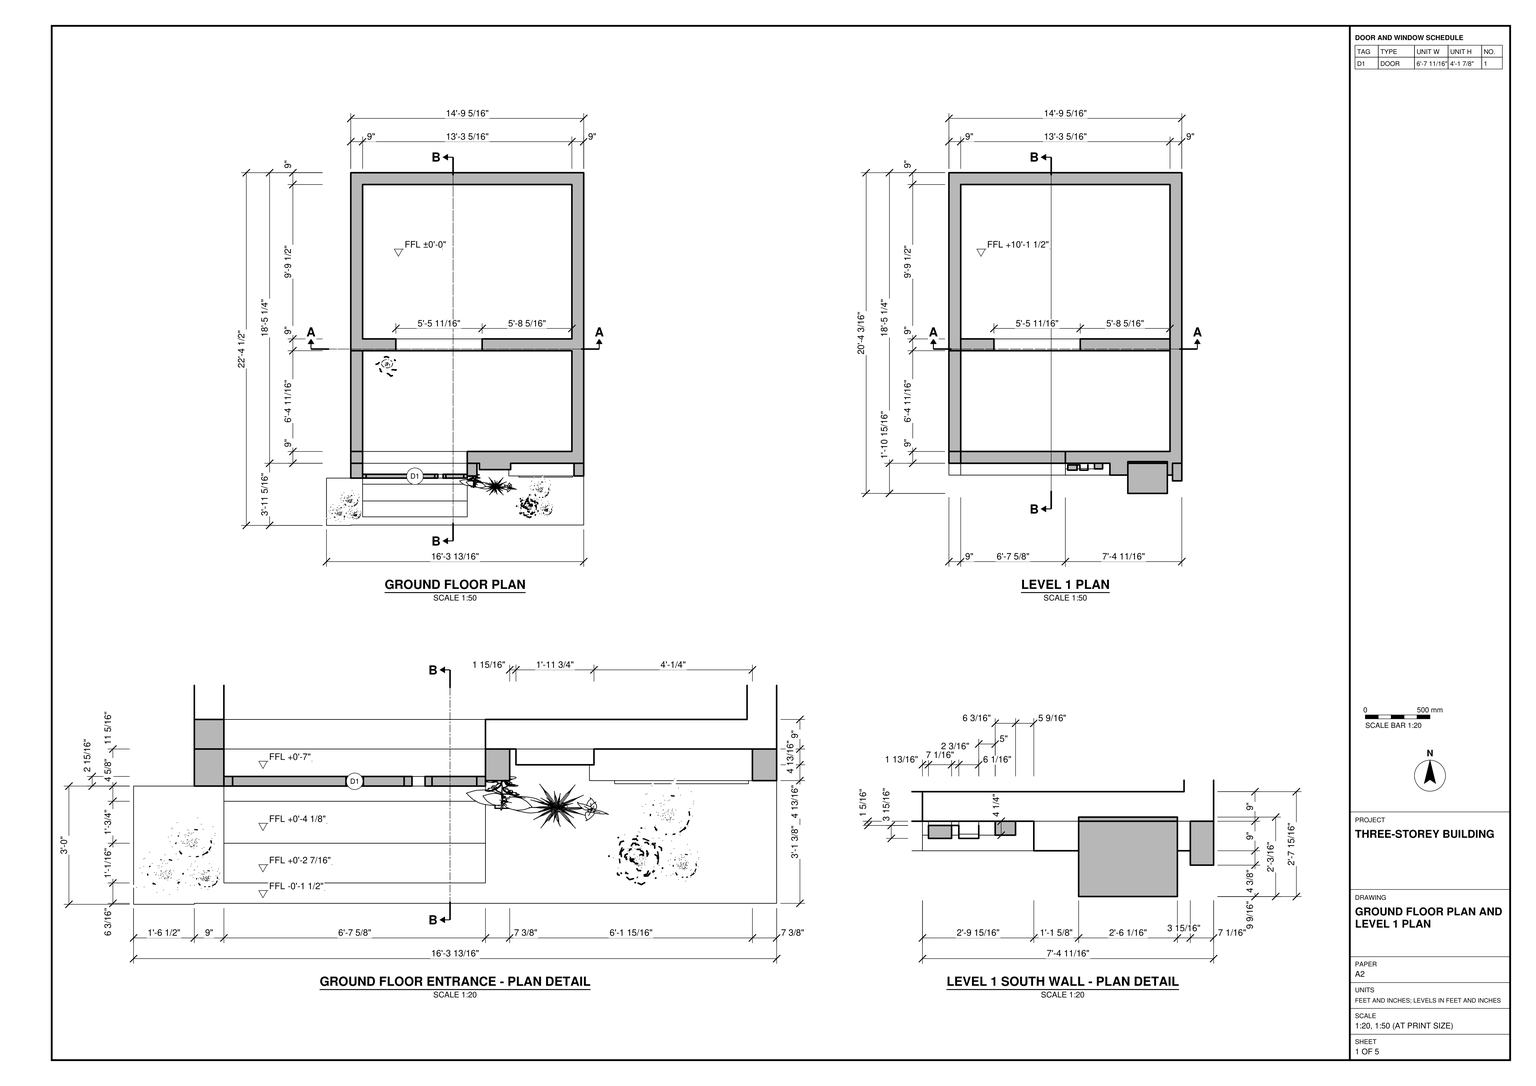
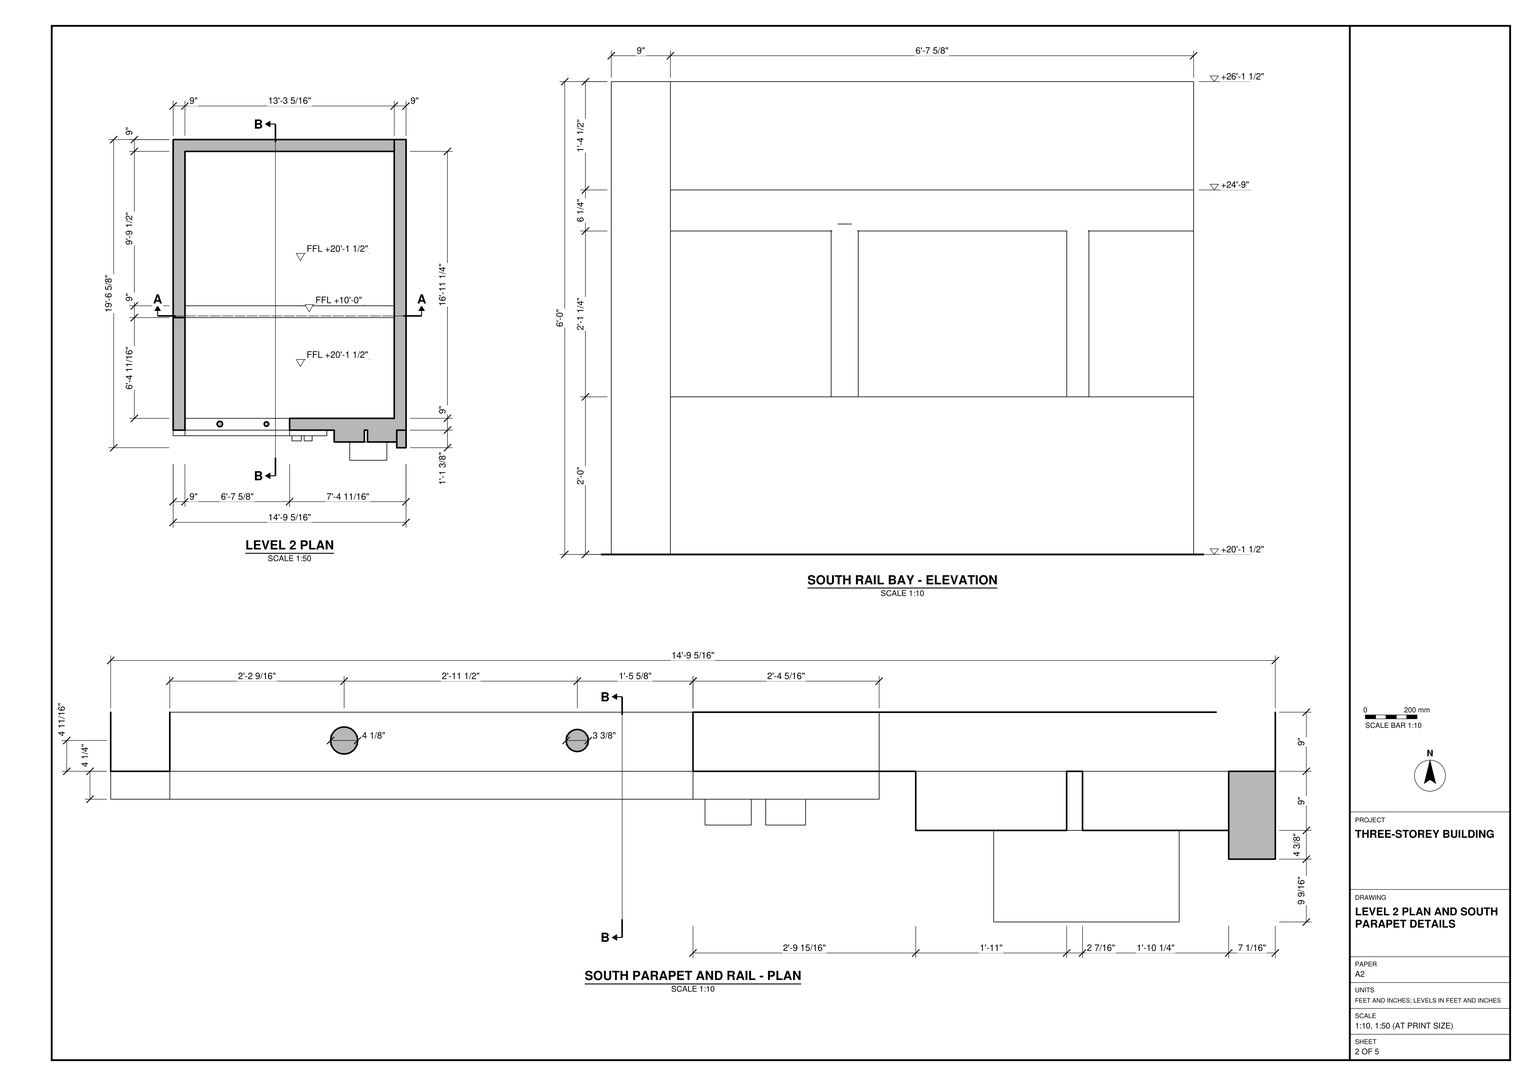
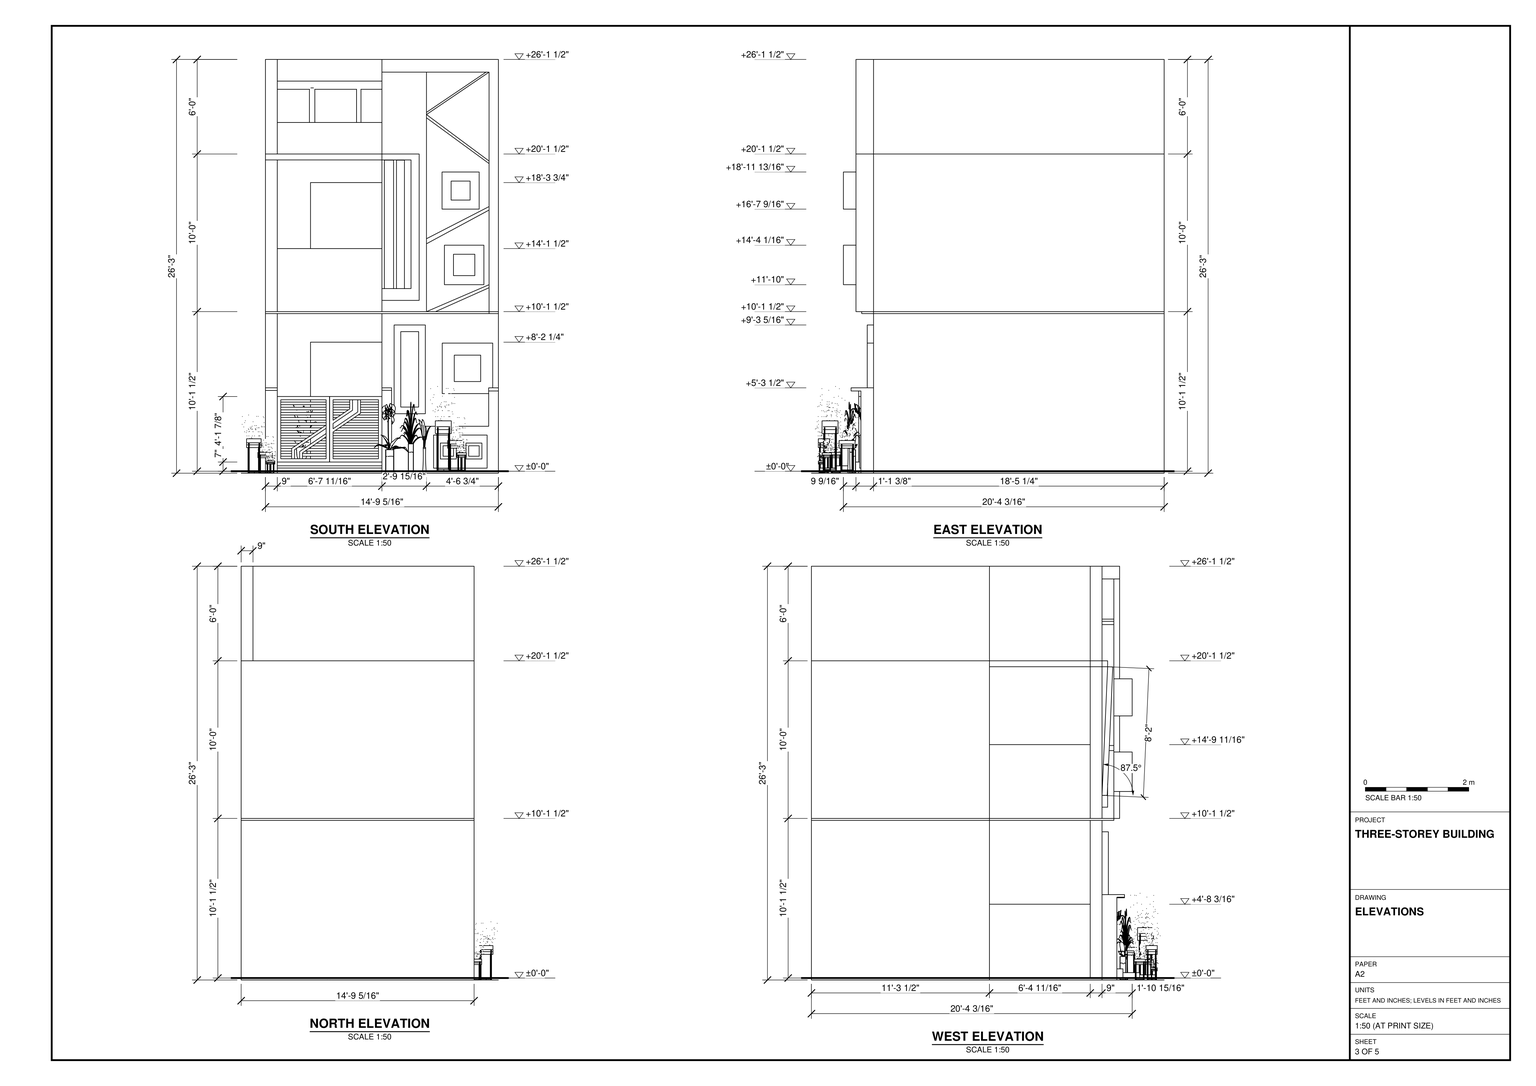
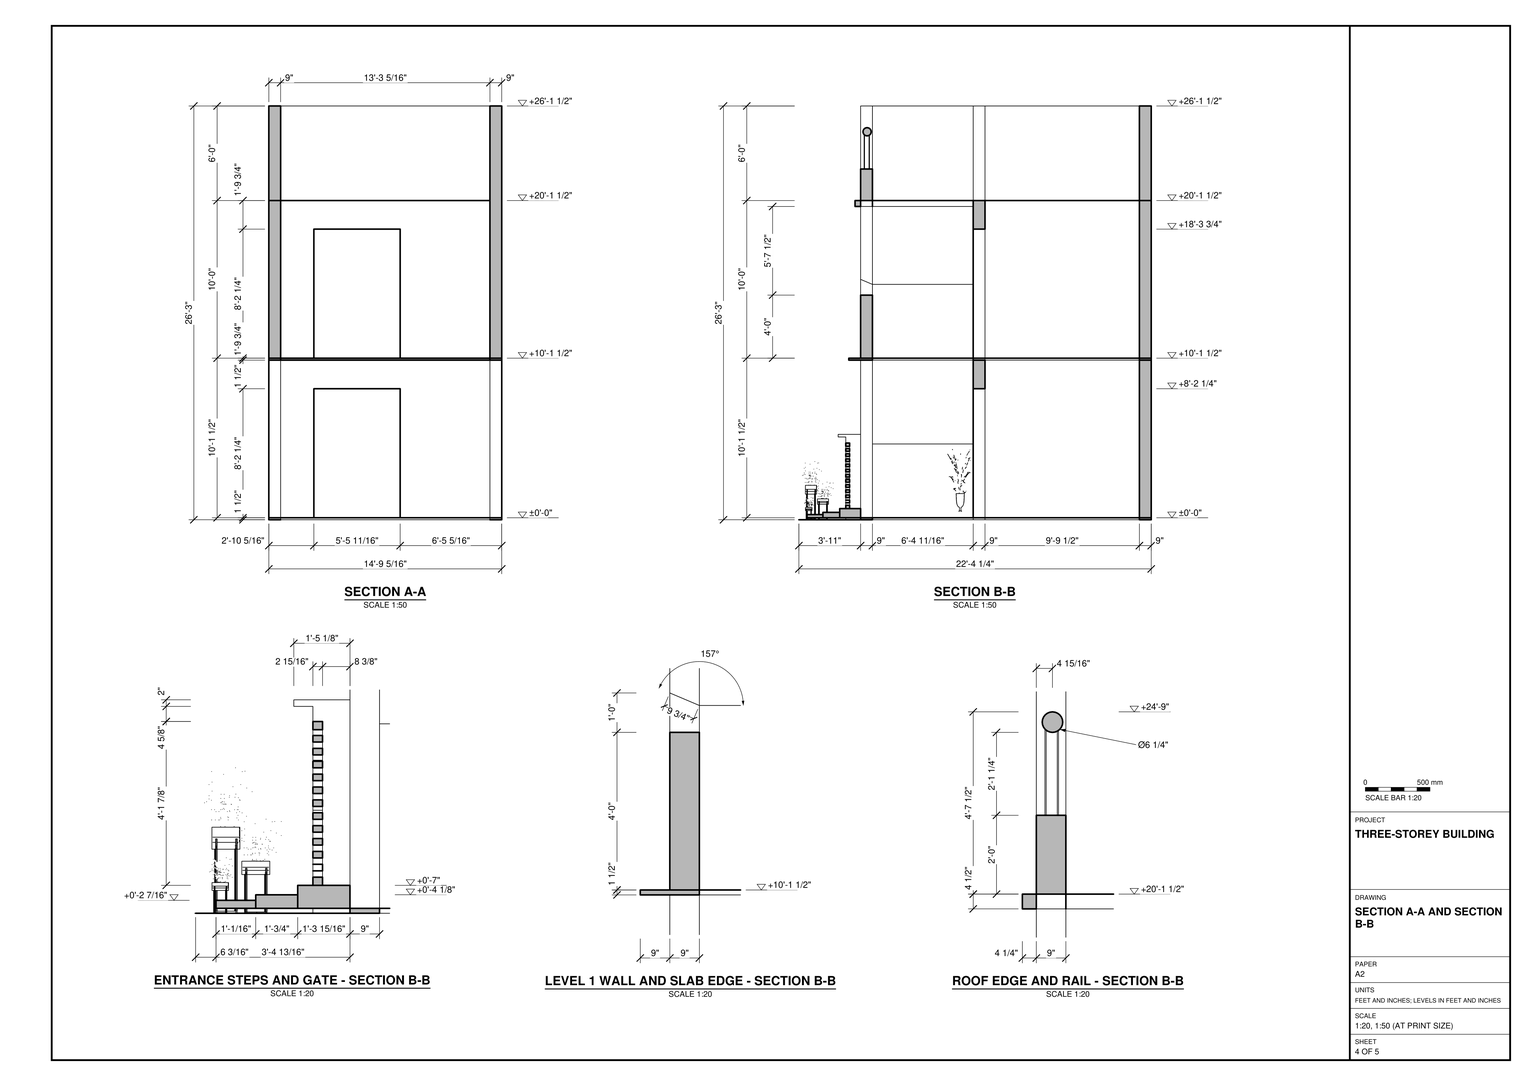
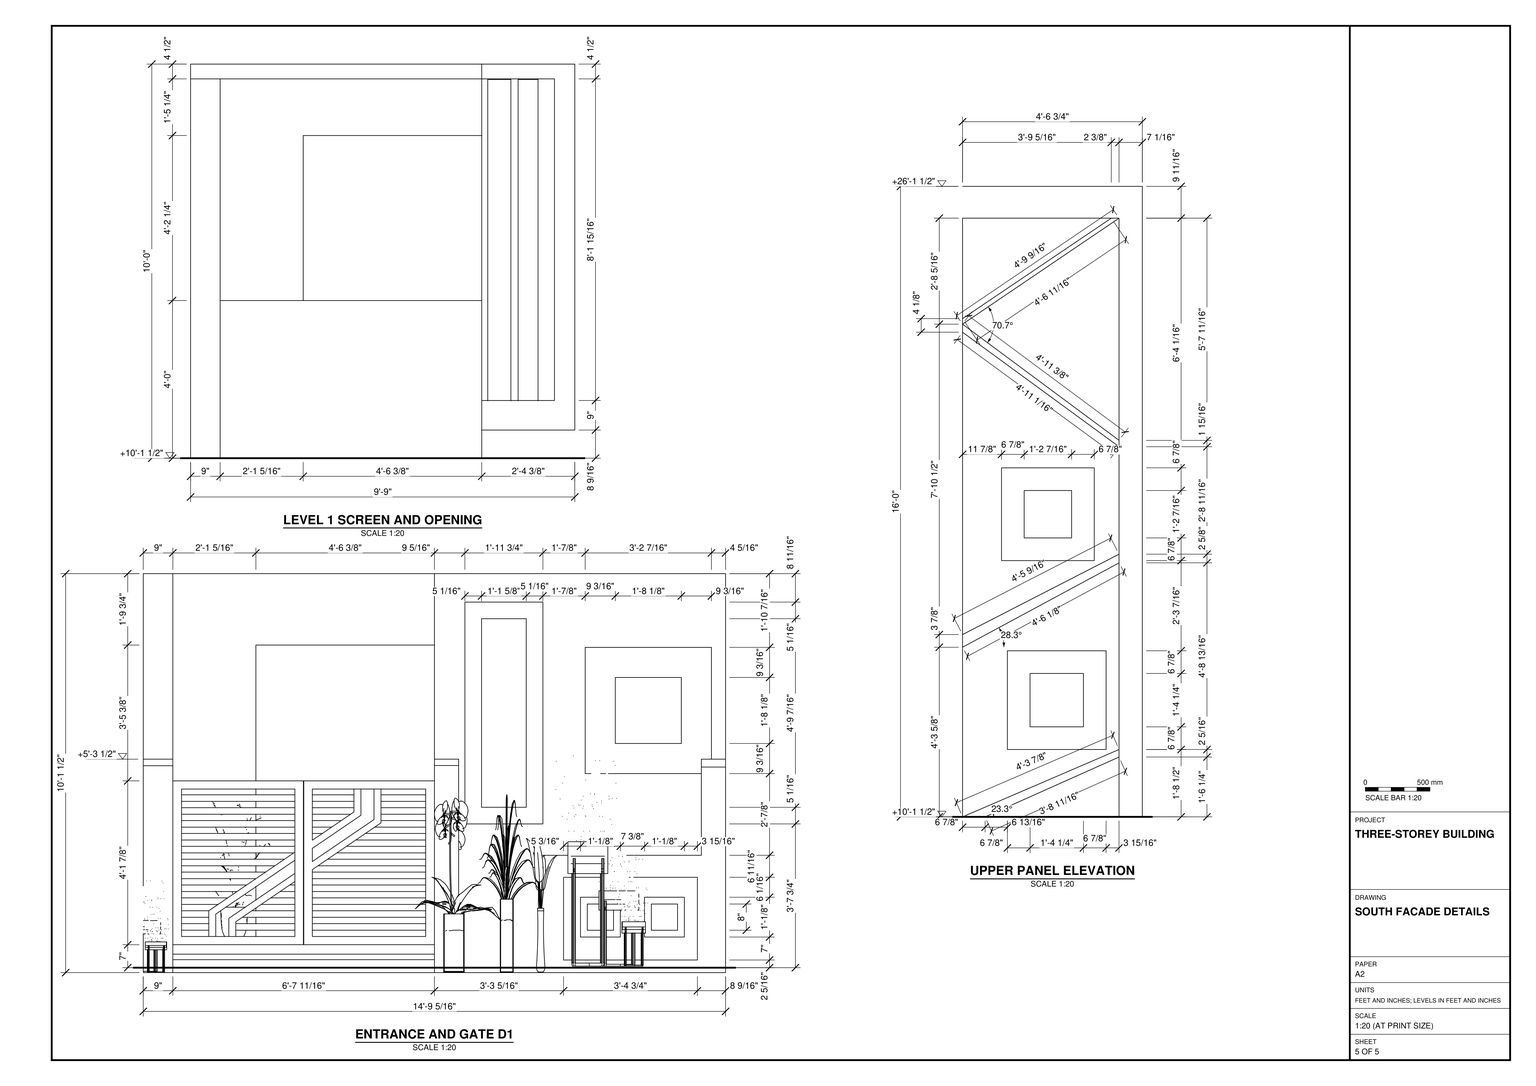
Build the three-storey building in SketchUp from task_files/diagram_01.pdf. Work in feet and inches. The overall model, including the entrance approach and façade projections, is 16'-6 7/8" wide, 22'-4 1/2" deep and 26'-3" high. Set the ground floor at ±0'-0", Level 1 at +10'-1 1/2" and Level 2 at +20'-1 1/2".

Use the plans to lay out the 9" walls and floor slabs. On the ground floor and Level 1, separate the deeper rear space from the shallower front space with a transverse wall, leaving the passage in the position shown. Finish Level 2 as a flat roof terrace with parapet walls and a divided rail bay on the south side.

Use the enlarged entrance plan to place the steps, landing and slatted gate on the left as seen in the south elevation. Align the recessed bay above the gate with the tall narrow façade panel beside it. Model the projecting square frames and diagonal bands on the right, while keeping the north and east walls plain. Decor and loose items, including the plants around the entrance, may be any suitable library components.

Keep walls, slabs, roof elements and individual furniture or joinery pieces in separate groups or components, and use components for repeated parts. Save one SketchUp model as output_files/three_storey_building_with_its_stepped_south_entrance.skp.

# SketchUp Ruby script. Lengths in inches.
U = 1.inch
M = Sketchup.active_model
def pt(a) = Geom::Point3d.new(a.map { |v| v * U })
def face(e, loops, mat)
  f = e.add_face(loops[0].map { |a| pt(a) })
  loops[1..].each { |l| e.add_face(l.map { |a| pt(a) }).erase! }
  f.material = f.back_material = mat if mat
  f
end
# faces: each face lists its corners as indices into pts; further lists are holes
def faces(e, pts, list, mat = nil) = list.each { |f| face(e, (f[0].is_a?(Array) ? f : [f]).map { |l| l.map { |i| pts[i] } }, mat) }
# xy, xz, yz: faces in a plane at the given z, y or x. An outline is a flat list of corners, or four numbers for a rectangle; further outlines are holes
def ring(l) = l.size == 4 ? [[l[0], l[1]], [l[2], l[1]], [l[2], l[3]], [l[0], l[3]]] : l.each_slice(2).to_a
def flat(e, list, mat, &to3) = list.each { |f| face(e, (f[0].is_a?(Array) ? f : [f]).map { |l| ring(l).map { |u, v| to3.(u, v) } }, mat) }
def xy(e, z, list, mat = nil) = flat(e, list, mat) { |x, y| [x, y, z] }
def xz(e, y, list, mat = nil) = flat(e, list, mat) { |x, z| [x, y, z] }
def yz(e, x, list, mat = nil) = flat(e, list, mat) { |y, z| [x, y, z] }
def lines(e, pts, list) = list.each { |a, b| e.add_line(pt(pts[a]), pt(pts[b])) }
# prism: a flat outline (further loops are holes) pulled along v
def prism(e, loops, v, mat = nil)
  f = face(e, loops, mat); d = Geom::Vector3d.new(v.map { |x| x * U })
  f.pushpull(f.normal.samedirection?(d) ? d.length : -d.length)
end
def box(e, o, s, mat = nil) = prism(e, [[o, [o[0] + s[0], o[1], o[2]], [o[0] + s[0], o[1] + s[1], o[2]], [o[0], o[1] + s[1], o[2]]]], [0, 0, s[2]], mat)
def at(x, y, z, deg = 0) = Geom::Transformation.translation(pt([x, y, z])) * Geom::Transformation.rotation(ORIGIN, Z_AXIS, deg.degrees)
def axes(o, x, y, z) = Geom::Transformation.new([*x, 0, *y, 0, *z, 0, *pt(o).to_a, 1])
def part(name) = M.definitions.add(name)
# library, detail: a bought-in or finely detailed component or shape, given as its bounding box
def library(name, o, s) = part(name).tap { |d| box(d.entities, o, s) }
def detail(e, o, s) = box(e.add_group.entities, o, s)
def put(e, d, t, mat = nil) = e.add_instance(d, t).tap { |i| i.material = mat if mat }
def group(e, t, mat = nil) = e.add_group.tap { |g| g.transformation = t; g.material = mat if mat }.entities
root = M.entities
M.materials.add("[Color B03]").color = [255, 140, 101]
M.materials.add("[Color B04]").color = [255, 101, 50]
M.materials.add("[Color B08]").color = [102, 25, 0]
M.materials.add("[Formica Speckled Grey]").color = [94, 105, 111]
M.materials.add("[Terrazzo Tile Light]").color = [219, 217, 210]
M.materials.add("[Translucent Glass Blue]").color = [100, 149, 237]
M.materials["[Translucent Glass Blue]"].alpha = 0.5
M.materials.add("[Translucent Glass Tinted]").color = [8, 201, 241]
M.materials["[Translucent Glass Tinted]"].alpha = 0.48
M.materials.add("[Wood Bamboo]").color = [177, 105, 43]
M.materials.add("[Wood Veneer 01]").color = [120, 70, 37]
c1 = library("plantas+internas",[0,0,0],[44.91,27.47,36.11])
c2 = library("blómastandur (1)",[6.48,-34.53,1.97],[34.7,40.11,68.37])
c3 = library("Decorative Plant",[-0.35,-0.24,0],[4.14,4.48,6.875])
c4 = library("Modern+Gate+1",[0,0,0],[118.11,1.97,78.74])
xy(root,-1.5,[[21.58,36,30.58,47.29],[110.23,37.67,117.61,47.29],[141.89,37.67,198.89,47.29],[21.58,47.29,198.89,47.29,198.89,268.51,21.58,268.51,21.58,132.99,30.58,132.99,30.58,259.51,189.89,259.51,189.89,56.29,30.58,56.29,30.58,132.99,21.58,132.99]])
xy(root,-1.5,[[3.08,0,21.58,0,21.58,0.29,198.89,0.29,198.89,37.67,141.89,37.67,141.89,47.29,117.61,47.29,117.61,37.67,110.23,37.67,110.23,47.29,30.58,47.29,30.58,36,3.08,36]],"[Formica Speckled Grey]")
xy(root,0,[[30.58,6.51,110.23,18.6],[30.58,18.6,110.23,31.37],[30.58,31.37,110.23,47.29],[110.23,47.29,110.23,56.29,189.89,56.29,189.89,132.99,121.56,132.99,121.56,141.99,189.89,141.99,189.89,259.51,30.58,259.51,30.58,141.99,55.87,141.99,55.87,132.99,21.58,132.99,21.58,268.51,198.89,268.51,198.89,47.29],[21.58,47.29,30.58,56.29],
  [30.58,47.29,110.23,56.29],[21.58,56.29,30.58,132.99],[30.58,56.29,189.89,132.99],[55.87,132.99,121.56,141.99],[30.58,141.99,189.89,259.51]])
xy(root,2.34,[[149.55,36.73,190.31,37.67]])
xy(root,2.4375,[[30.58,6.51,110.23,18.6]],"[Terrazzo Tile Light]")
xy(root,4.125,[[30.58,18.6,110.23,31.37]],"[Terrazzo Tile Light]")
xy(root,7,[[30.58,31.37,110.23,47.29]],"[Terrazzo Tile Light]")
xy(root,9.33,[[154.72,36.73,166.84,37.67],[174.22,36.73,186.34,37.67]])
xy(root,21.45,[[154.72,36.73,166.84,37.67],[174.22,36.73,186.34,37.67]])
xy(root,27.52,[[149.55,36.73,190.31,37.67]])
xy(root,34.22,[[141.89,37.67,191.52,47.29]],"[Color B04]")
xy(root,43.77,[[119.52,42.48,143.27,47.29]])
xy(root,48.84,[[124.59,42.48,138.2,47.29]])
xy(root,56.1875,[[21.58,56.29,30.58,132.99]],"[Color B04]")
xy(root,59.11,[[156.15,42.48,194.58,47.29]],"[Color B03]")
xy(root,61.09,[[191.52,30.1875,198.89,37.67]])
xy(root,61.5,[[21.58,30.1875,30.58,36]])
xy(root,61.5625,[[110.23,30.1875,117.61,37.67]])
xy(root,63.5,[[21.58,30.1875,30.58,47.29],[110.23,30.1875,117.61,47.29],[191.52,30.1875,198.89,47.29]],"[Color B04]")
xy(root,68.27,[[165.31,42.48,185.42,47.29]])
xy(root,88.375,[[165.31,42.48,185.42,47.29]])
xy(root,97.54,[[156.15,42.48,194.58,47.29]],"[Color B03]")
xy(root,98.25,[[55.87,132.99,121.56,141.99]])
xy(root,106.27,[[124.59,42.48,138.2,47.29]])
xy(root,111.34,[[119.52,42.48,143.27,47.29]])
xy(root,120,[[21.58,38.29,30.58,47.29],[30.58,38.29,110.23,56.29],[110.23,38.29,191.8,47.29],[110.23,47.29,198.89,47.29,198.89,268.51,21.58,268.51,21.58,132.99,30.58,132.99,30.58,259.51,189.89,259.51,189.89,56.29,110.23,56.29],[21.58,47.29,30.58,56.29],
  [21.58,56.29,30.58,132.99],[30.58,132.99,189.89,141.99]])
xy(root,121.5,[[191.8,33.92,198.89,47.29],[151.02,38.29,151.02,47.29,110.23,47.29,110.23,56.29,189.89,56.29,189.89,132.99,121.56,132.99,121.56,141.99,189.89,141.99,189.89,259.51,30.58,259.51,30.58,141.99,55.87,141.99,55.87,132.99,21.58,132.99,21.58,268.51,198.89,268.51,198.89,47.29,191.8,47.29,191.8,38.29],[144.15,38.29,151.02,47.29],[21.58,47.29,30.58,56.29],[30.58,47.29,110.23,56.29],
  [21.58,56.29,30.58,132.99],[30.58,56.29,189.89,132.99],[55.87,132.99,121.56,141.99],[30.58,141.99,189.89,259.51]])
xy(root,121.5,[[21.58,38.29,30.58,47.29],[30.58,38.29,110.23,47.29],[110.23,38.29,144.15,47.29]],"[Color B04]")
xy(root,130.0625,[[110.23,43.04,138.58,47.29]])
xy(root,139.0625,[[110.23,43.04,132.38,47.29]])
xy(root,142.02,[[157.8,24.35,187.86,38.29],[157.8,38.29,187.86,47.29],[157.8,47.29,187.86,48.54]])
xy(root,148.92,[[164.7,47.29,180.96,48.54]])
xy(root,148.92,[[164.7,24.35,180.96,47.29]],"[Color B08]")
xy(root,165.18,[[164.7,47.29,180.96,48.54]])
xy(root,165.18,[[164.7,24.35,180.96,47.29]],"[Color B08]")
xy(root,169.5,[[30.58,47.29,110.23,56.29]])
xy(root,172.08,[[157.8,24.35,187.86,38.29],[157.8,38.29,187.86,47.29],[157.8,47.29,187.86,48.54]])
xy(root,177.6875,[[21.58,56.29,30.58,132.99]],"[Color B04]")
xy(root,199.54,[[156.01,24.35,184.26,38.29],[156.01,38.29,184.26,47.29]])
xy(root,206.44,[[162.91,24.35,177.36,47.29]],"[Color B08]")
xy(root,219.75,[[55.87,132.99,121.56,141.99]])
xy(root,220.89,[[162.91,24.35,177.36,47.29]],"[Color B08]")
xy(root,227.79,[[156.01,24.35,184.26,38.29],[156.01,38.29,184.26,47.29]])
xy(root,237,[[21.58,43.04,30.58,47.29],[30.58,43.04,110.23,47.29],[110.23,43.04,132.38,47.29],[21.58,47.29,30.58,132.99]])
xy(root,241.5,[[21.58,43.04,30.58,47.29],[30.58,43.04,110.23,47.29],[110.23,43.04,138.58,47.29],[21.58,47.29,30.58,132.99],[30.58,47.29,110.23,56.29],
  [110.23,47.29,138.58,56.29],[30.58,56.29,189.89,132.99],[21.58,132.99,21.58,268.51,189.89,268.51,189.89,259.51,30.58,259.51,30.58,132.99],[30.58,132.99,189.89,141.99],[30.58,141.99,189.89,259.51]])
xy(root,265.5,[[[30.58,47.29,110.23,56.29],[57.11,49.92,56.58,49.99,56.08,50.2,55.66,50.52,55.33,50.95,55.12,51.45,55.05,51.98,55.12,52.52,55.33,53.01,55.66,53.44,56.08,53.77,56.58,53.98,57.11,54.05,57.65,53.98,58.15,53.77,58.57,53.44,58.9,53.01,59.11,52.52,59.18,51.98,59.11,51.45,58.9,50.95,58.57,50.52,58.15,50.2,57.65,49.99],[92.61,50.3,92.17,50.35,91.77,50.52,91.42,50.79,91.15,51.14,90.98,51.55,90.92,51.98,90.98,52.42,91.15,52.83,91.42,53.18,91.77,53.44,92.17,53.61,92.61,53.67,93.05,53.61,93.45,53.44,93.8,53.18,94.07,52.83,94.24,52.42,94.3,51.98,94.24,51.55,94.07,51.14,93.8,50.79,93.45,50.52,93.05,50.35]]])
xy(root,291.8125,[[57.11,49.92,57.65,49.99,58.15,50.2,58.57,50.52,58.9,50.95,59.11,51.45,59.18,51.98,59.11,52.52,58.9,53.01,58.57,53.44,58.15,53.77,57.65,53.98,57.11,54.05,56.58,53.98,56.08,53.77,55.66,53.44,55.33,53.01,55.12,52.52,55.05,51.98,55.12,51.45,55.33,50.95,55.66,50.52,56.08,50.2,56.58,49.99]])
xy(root,292.875,[[92.61,50.3,93.05,50.35,93.45,50.52,93.8,50.79,94.07,51.14,94.24,51.55,94.3,51.98,94.24,52.42,94.07,52.83,93.8,53.18,93.45,53.44,93.05,53.61,92.61,53.67,92.17,53.61,91.77,53.44,91.42,53.18,91.15,52.83,90.98,52.42,90.92,51.98,90.98,51.55,91.15,51.14,91.42,50.79,91.77,50.52,92.17,50.35]])
xy(root,303.82,[[110.23,33.92,144.15,47.29],[144.15,33.92,144.15,38.29,189.45,38.29,189.45,47.29,191.8,47.29,191.8,33.92],[144.15,38.29,189.45,47.29]])
xy(root,313.5,[[110.23,33.92,198.89,47.29],[21.58,47.29,30.58,132.99],[21.58,132.99,30.58,132.99,30.58,259.51,189.89,259.51,189.89,268.51,21.58,268.51]])
xy(root,313.5,[[110.23,47.29,198.89,47.29,198.89,268.51,189.89,268.51,189.89,56.29,110.23,56.29]],"[Formica Speckled Grey]")
xz(root,6.51,[[30.58,0,110.23,2.4375]],"[Terrazzo Tile Light]")
xz(root,18.6,[[30.58,0,110.23,2.4375]])
xz(root,18.6,[[30.58,2.4375,110.23,4.125]],"[Terrazzo Tile Light]")
xz(root,24.35,[[[157.8,142.02,187.86,172.08],[164.7,148.92,180.96,165.18]],[[156.01,199.54,184.26,227.79],[162.91,206.44,177.36,220.89]]])
xz(root,30.1875,[[191.52,61.09,198.89,63.5],[21.58,61.5,30.58,63.5],[110.23,61.5625,117.61,63.5]],"[Color B04]")
xz(root,31.37,[[30.58,0,110.23,4.125]])
xz(root,31.37,[[30.58,4.125,110.23,7]],"[Terrazzo Tile Light]")
xz(root,33.92,[[191.8,121.5,198.89,121.5,198.89,313.5,110.23,313.5,110.23,303.82,191.8,303.82]],"[Color B04]")
xz(root,36,[[21.58,-1.5,30.58,61.5]],"[Color B04]")
xz(root,36.73,[[[149.55,2.34,190.31,27.52],[154.72,9.33,166.84,21.45],[174.22,9.33,186.34,21.45]]],"[Color B08]")
xz(root,37.67,[[[149.55,2.34,190.31,27.52],[154.72,9.33,166.84,21.45],[174.22,9.33,186.34,21.45]],[[154.72,9.33,166.84,21.45],[156.79,11.4,164.77,19.38]],[[174.22,9.33,186.34,21.45],[176.29,11.4,184.27,19.38]]])
xz(root,37.67,[[110.23,-1.5,117.61,61.5625],[[141.89,-1.5,198.89,-1.5,198.89,61.09,191.52,61.09,191.52,34.22,141.89,34.22],[149.55,2.34,190.31,27.52]]],"[Color B04]")
xz(root,37.67,[[156.79,11.4,164.77,19.38],[176.29,11.4,184.27,19.38]],"[Color B08]")
xz(root,38.29,[[21.58,120,191.8,121.5]],"[Color B04]")
xz(root,38.29,[[[144.15,121.5,191.8,142.02,191.8,198.85,144.15,173.17],[157.8,142.02,187.86,172.08]],[151.02,121.5,191.8,121.5,191.8,139.72],[[144.15,177.02,191.8,201.49,191.8,234.22,144.15,269.08],[156.01,199.54,184.26,227.79]],[191.8,236.16,191.8,303.82,144.15,271.54],[144.15,273.23,189.45,303.82,144.15,303.82]],"[Color B08]")
xz(root,42.48,[[[119.52,43.77,143.27,111.34],[124.59,48.84,138.2,106.27]]])
xz(root,42.48,[[[156.15,59.11,194.58,97.54],[165.31,68.27,185.42,88.375]]],"[Color B03]")
xz(root,43.04,[[110.23,130.0625,138.58,130.0625,138.58,241.5,110.23,241.5,110.23,237,132.38,237,132.38,139.0625,110.23,139.0625],[21.58,237,110.23,241.5]],"[Color B04]")
xz(root,47.29,[[21.58,-1.5,30.58,0],[30.58,-1.5,110.23,0],[110.23,-1.5,117.61,0],[117.61,-1.5,141.89,0],[141.89,-1.5,198.89,0],
  [21.58,0,30.58,63.5],[30.58,0,110.23,7],[191.52,59.11,194.58,63.5],[165.31,68.27,185.42,88.375],[191.8,120,198.89,121.5],
  [191.8,121.5,191.8,303.82,110.23,303.82,110.23,313.5,198.89,313.5,198.89,121.5],[144.15,121.5,151.02,121.5,191.8,139.72,191.8,142.02],[110.23,130.0625,110.23,139.0625,132.38,139.0625,132.38,237,110.23,237,110.23,241.5,138.58,241.5,138.58,130.0625],[[157.8,142.02,187.86,172.08],[164.7,148.92,180.96,165.18]],[144.15,173.17,191.8,198.85,191.8,201.49,144.15,177.02],
  [[156.01,199.54,184.26,227.79],[162.91,206.44,177.36,220.89]],[191.8,234.22,191.8,236.16,144.15,271.54,144.15,269.08],[21.58,237,110.23,241.5],[144.15,271.54,191.8,303.82,189.45,303.82,144.15,273.23]])
xz(root,47.29,[[21.58,63.5,30.58,120],[21.58,121.5,30.58,237],[110.23,121.5,144.15,121.5,144.15,303.82,110.23,303.82,110.23,241.5,138.58,241.5,138.58,130.0625,110.23,130.0625],[21.58,241.5,30.58,313.5],[30.58,241.5,110.23,265.5]],"[Color B04]")
xz(root,47.29,[[110.23,0,117.61,63.5],[[117.61,0,141.89,0,141.89,34.22,191.52,34.22,191.52,59.11,156.15,59.11,156.15,97.54,194.58,97.54,194.58,63.5,198.89,63.5,198.89,120,110.23,120,110.23,63.5,117.61,63.5],[119.52,43.77,143.27,111.34]],[141.89,0,198.89,0,198.89,63.5,194.58,63.5,194.58,59.11,191.52,59.11,191.52,34.22,141.89,34.22],[164.7,148.92,180.96,165.18],[162.91,206.44,177.36,220.89]],"[Color B08]")
xz(root,47.29,[[30.58,121.5,110.23,169.5]],"[Translucent Glass Blue]")
xz(root,47.29,[[124.59,48.84,138.2,106.27]],"[Translucent Glass Tinted]")
xz(root,47.29,[[110.23,139.0625,132.38,237]],"[Wood Bamboo]")
xz(root,48.54,[[[157.8,142.02,187.86,172.08],[164.7,148.92,180.96,165.18]]])
xz(root,56.29,[[30.58,-1.5,189.89,0],[21.58,0,30.58,56.1875],[110.23,0,189.89,120],[21.58,56.1875,30.58,120],[30.58,120,189.89,121.5],
  [21.58,121.5,30.58,177.6875],[30.58,121.5,110.23,169.5],[110.23,121.5,110.23,237,138.58,237,138.58,241.5,189.89,241.5,189.89,121.5],[30.58,237,110.23,241.5],[110.23,237,138.58,241.5],
  [30.58,241.5,110.23,265.5],[110.23,241.5,189.89,313.5]])
xz(root,132.99,[[21.58,-1.5,30.58,0],[21.58,0,30.58,56.1875],[21.58,120,30.58,121.5],[30.58,120,189.89,121.5],[21.58,121.5,30.58,177.6875],
  [21.58,237,30.58,241.5],[21.58,241.5,30.58,313.5]])
xz(root,132.99,[[30.58,0,55.87,0,55.87,98.25,121.56,98.25,121.56,0,189.89,0,189.89,120,30.58,120],[21.58,56.1875,30.58,120],[30.58,121.5,55.87,121.5,55.87,219.75,121.56,219.75,121.56,121.5,189.89,121.5,189.89,241.5,30.58,241.5],[21.58,177.6875,30.58,237]],"[Color B04]")
xz(root,132.99,[[55.87,0,121.56,98.25],[55.87,121.5,121.56,219.75]],"[Wood Veneer 01]")
xz(root,141.99,[[30.58,0,30.58,120,189.89,120,189.89,0,121.56,0,121.56,98.25,55.87,98.25,55.87,0],[30.58,121.5,30.58,241.5,189.89,241.5,189.89,121.5,121.56,121.5,121.56,219.75,55.87,219.75,55.87,121.5]])
xz(root,259.51,[[30.58,-1.5,189.89,0],[30.58,0,189.89,120],[30.58,120,189.89,121.5],[30.58,121.5,189.89,241.5]])
xz(root,259.51,[[30.58,241.5,189.89,313.5]],"[Formica Speckled Grey]")
xz(root,268.51,[[21.58,-1.5,198.89,0],[21.58,120,198.89,121.5]])
xz(root,268.51,[[21.58,0,198.89,120],[21.58,121.5,198.89,241.5],[21.58,241.5,189.89,313.5],[189.89,241.5,198.89,313.5]],"[Terrazzo Tile Light]")
yz(root,21.58,[[47.29,-1.5,132.99,0],[132.99,-1.5,268.51,0],[38.29,120,132.99,121.5],[132.99,120,268.51,121.5],[43.04,237,47.29,241.5],
  [47.29,237,56.29,241.5],[56.29,237,132.99,241.5]])
yz(root,21.58,[[36,-1.5,36,61.5,30.1875,61.5,30.1875,63.5,47.29,63.5,47.29,-1.5],[47.29,0,56.29,120],[56.29,0,132.99,56.1875],[47.29,121.5,56.29,237]],"[Color B04]")
yz(root,21.58,[[132.99,0,268.51,120],[132.99,121.5,268.51,241.5],[47.29,241.5,56.29,313.5],[56.29,241.5,132.99,313.5],[132.99,241.5,268.51,313.5]],"[Terrazzo Tile Light]")
yz(root,21.58,[[56.29,121.5,132.99,177.6875]],"[Translucent Glass Blue]")
yz(root,30.58,[[36,-1.5,47.29,0],[56.29,-1.5,132.99,0],[141.99,-1.5,259.51,0],[6.51,0,18.6,2.4375],[18.6,0,31.37,4.125],
  [31.37,0,36,7],[36,0,47.29,7],[141.99,0,259.51,120],[56.29,120,132.99,121.5],[132.99,120,141.99,241.5],
  [141.99,120,259.51,121.5],[47.29,121.5,56.29,169.5],[141.99,121.5,259.51,241.5],[56.29,237,132.99,241.5],[47.29,241.5,56.29,265.5],
  [132.99,241.5,141.99,313.5]])
yz(root,30.58,[[47.29,0,56.29,120],[56.29,0,132.99,56.1875],[36,7,47.29,7,47.29,63.5,30.1875,63.5,30.1875,61.5,36,61.5],[56.29,121.5,132.99,177.6875],[47.29,169.5,56.29,169.5,56.29,177.6875,47.29,181.5],
  [56.29,177.6875,56.29,237,47.29,237,47.29,181.5]],"[Color B04]")
yz(root,30.58,[[56.29,241.5,132.99,313.5],[141.99,241.5,259.51,313.5],[[47.29,265.5,56.29,313.5],[52.21,290.75,51.4,290.86,50.65,291.17,50,291.67,49.5,292.32,49.19,293.07,49.08,293.88,49.19,294.6875,49.5,295.44,50,296.09,50.65,296.58,51.4,296.9,52.21,297,53.02,296.9,53.77,296.58,54.42,296.09,54.91,295.44,55.23,294.6875,55.33,293.88,55.23,293.07,54.91,292.32,54.42,291.67,53.77,291.17,53.02,290.86]]],"[Formica Speckled Grey]")
yz(root,55.87,[[132.99,0,141.99,98.25],[132.99,121.5,141.99,219.75]])
yz(root,110.23,[[37.67,-1.5,47.29,0],[6.51,0,18.6,2.4375],[18.6,0,31.37,4.125],[31.37,0,37.67,7],[37.67,0,47.29,7],
  [47.29,121.5,56.29,169.5],[43.04,130.0625,47.29,139.0625],[47.29,169.5,56.29,241.5],[43.04,237,47.29,241.5],[47.29,241.5,56.29,265.5],
  [47.29,265.5,56.29,313.5],[33.92,303.82,47.29,313.5]])
yz(root,110.23,[[47.29,0,56.29,120],[37.67,7,37.67,61.5625,30.1875,61.5625,30.1875,63.5,47.29,63.5,47.29,7]],"[Color B04]")
yz(root,110.39,[[52.21,290.75,53.02,290.86,53.77,291.17,54.42,291.67,54.91,292.32,55.23,293.07,55.33,293.88,55.23,294.6875,54.91,295.44,54.42,296.09,53.77,296.58,53.02,296.9,52.21,297,51.4,296.9,50.65,296.58,50,296.09,49.5,295.44,49.19,294.6875,49.08,293.88,49.19,293.07,49.5,292.32,50,291.67,50.65,291.17,51.4,290.86]])
yz(root,112.07,[[43.36,138.89,39.11,236.83,43.04,237,47.29,139.0625]],"[Wood Bamboo]")
yz(root,117.61,[[37.67,-1.5,47.29,-1.5,47.29,63.5,30.1875,63.5,30.1875,61.5625,37.67,61.5625]],"[Color B04]")
yz(root,119.11,[[43.36,138.89,47.29,139.0625,43.04,237,39.11,236.83]])
yz(root,119.52,[[42.48,43.77,47.29,111.34]])
yz(root,121.31,[[43.36,138.89,39.11,236.83,43.04,237,47.29,139.0625]],"[Wood Bamboo]")
yz(root,121.56,[[132.99,0,141.99,98.25],[132.99,121.5,141.99,219.75]])
yz(root,124.59,[[42.48,48.84,47.29,106.27]])
yz(root,127.375,[[43.36,138.89,47.29,139.0625,43.04,237,39.11,236.83]],"[Wood Bamboo]")
yz(root,132.38,[[43.04,139.0625,47.29,237]])
yz(root,138.2,[[42.48,48.84,47.29,106.27]])
yz(root,138.58,[[43.04,130.0625,47.29,237],[43.04,237,47.29,241.5],[47.29,237,56.29,241.5]])
yz(root,141.89,[[37.67,-1.5,47.29,34.22]],"[Color B04]")
yz(root,143.27,[[42.48,43.77,47.29,111.34]])
yz(root,144.15,[[38.29,121.5,47.29,173.17],[38.29,177.02,47.29,269.08],[38.29,273.23,47.29,303.82]],"[Color B08]")
yz(root,149.55,[[36.73,2.34,37.67,27.52]])
yz(root,154.72,[[36.73,9.33,37.67,21.45]])
yz(root,156.01,[[24.35,199.54,38.29,227.79],[38.29,199.54,47.29,227.79]])
yz(root,156.15,[[42.48,59.11,47.29,97.54]],"[Color B03]")
yz(root,157.8,[[24.35,142.02,38.29,172.08],[38.29,142.02,47.29,172.08],[47.29,142.02,48.54,172.08]])
yz(root,162.91,[[24.35,206.44,47.29,220.89]],"[Color B08]")
yz(root,164.7,[[47.29,148.92,48.54,165.18]])
yz(root,164.7,[[24.35,148.92,47.29,165.18]],"[Color B08]")
yz(root,165.31,[[42.48,68.27,47.29,88.375]])
yz(root,166.84,[[36.73,9.33,37.67,21.45]])
yz(root,174.22,[[36.73,9.33,37.67,21.45]])
yz(root,177.36,[[24.35,206.44,47.29,220.89]],"[Color B08]")
yz(root,180.96,[[47.29,148.92,48.54,165.18]])
yz(root,180.96,[[24.35,148.92,47.29,165.18]],"[Color B08]")
yz(root,184.26,[[24.35,199.54,38.29,227.79],[38.29,199.54,47.29,227.79]])
yz(root,185.42,[[42.48,68.27,47.29,88.375]])
yz(root,186.34,[[36.73,9.33,37.67,21.45]])
yz(root,187.86,[[24.35,142.02,38.29,172.08],[38.29,142.02,47.29,172.08],[47.29,142.02,48.54,172.08]])
yz(root,189.89,[[56.29,-1.5,132.99,0],[141.99,-1.5,259.51,0],[56.29,0,132.99,120],[141.99,0,259.51,120],[56.29,120,132.99,121.5],
  [132.99,120,141.99,241.5],[141.99,120,259.51,121.5],[56.29,121.5,132.99,241.5],[141.99,121.5,259.51,241.5],[132.99,241.5,141.99,313.5],
  [259.51,241.5,268.51,313.5]])
yz(root,189.89,[[56.29,241.5,132.99,313.5],[141.99,241.5,259.51,313.5]],"[Formica Speckled Grey]")
yz(root,190.31,[[36.73,2.34,37.67,27.52]])
yz(root,191.52,[[37.67,34.22,37.67,61.09,30.1875,61.09,30.1875,63.5,47.29,63.5,47.29,34.22]],"[Color B04]")
yz(root,191.8,[[38.29,120,47.29,121.5],[33.92,121.5,33.92,303.82,38.29,303.82,38.29,236.16,47.29,236.16,47.29,234.22,38.29,234.22,38.29,201.49,47.29,201.49,47.29,198.85,38.29,198.85,38.29,142.02,47.29,142.02,47.29,139.72,38.29,139.72,38.29,121.5],[38.29,121.5,47.29,139.72],[38.29,142.02,47.29,198.85],[38.29,142.02,47.29,198.85],
  [38.29,201.49,47.29,234.22],[38.29,236.16,47.29,303.82]])
yz(root,194.58,[[42.48,59.11,47.29,97.54]],"[Color B03]")
yz(root,198.89,[[47.29,-1.5,268.51,0],[47.29,120,268.51,121.5]])
yz(root,198.89,[[37.67,-1.5,47.29,-1.5,47.29,63.5,30.1875,63.5,30.1875,61.09,37.67,61.09],[33.92,121.5,47.29,241.5],[33.92,241.5,47.29,313.5]],"[Color B04]")
yz(root,198.89,[[47.29,0,268.51,120],[47.29,121.5,268.51,241.5],[47.29,241.5,268.51,313.5]],"[Terrazzo Tile Light]")
p = [[144.15,47.29,121.5],[191.8,47.29,142.02],[191.8,38.29,142.02],[144.15,38.29,121.5],[191.8,47.29,139.72],[151.02,47.29,121.5],
  [151.02,38.29,121.5],[191.8,38.29,139.72],[112.07,39.11,236.83],[112.07,43.36,138.89],[119.11,43.36,138.89],[119.11,39.11,236.83],
  [121.31,39.11,236.83],[121.31,43.36,138.89],[127.375,43.36,138.89],[127.375,39.11,236.83],[112.07,47.29,139.0625],[119.11,47.29,139.0625],
  [121.31,47.29,139.0625],[127.375,47.29,139.0625],[112.07,43.04,237],[119.11,43.04,237],[121.31,43.04,237],[191.8,47.29,198.85],
  [144.15,47.29,173.17],[144.15,38.29,173.17],[191.8,38.29,198.85],[144.15,47.29,177.02],[191.8,47.29,201.49],[191.8,38.29,201.49],
  [144.15,38.29,177.02],[191.8,47.29,234.22],[144.15,47.29,269.08],[144.15,38.29,269.08],[191.8,38.29,234.22],[144.15,47.29,271.54],
  [191.8,47.29,236.16],[191.8,38.29,236.16],[144.15,38.29,271.54],[127.375,43.04,237],[56.58,49.99,265.5],[57.11,49.92,265.5],
  [57.11,49.92,291.8125],[56.58,49.99,291.8125],[57.65,49.99,265.5],[57.65,49.99,291.8125],[56.08,50.2,265.5],[56.08,50.2,291.8125],
  [58.15,50.2,265.5],[58.15,50.2,291.8125],[55.66,50.52,265.5],[55.66,50.52,291.8125],[58.57,50.52,265.5],[58.57,50.52,291.8125],
  [92.17,50.35,265.5],[92.61,50.3,265.5],[92.61,50.3,292.875],[92.17,50.35,292.875],[93.05,50.35,265.5],[93.05,50.35,292.875],
  [91.77,50.52,265.5],[91.77,50.52,292.875],[93.45,50.52,265.5],[93.45,50.52,292.875],[55.33,50.95,265.5],[55.33,50.95,291.8125],
  [58.9,50.95,265.5],[58.9,50.95,291.8125],[91.42,50.79,265.5],[91.42,50.79,292.875],[93.8,50.79,265.5],[93.8,50.79,292.875],
  [91.15,51.14,265.5],[91.15,51.14,292.875],[94.07,51.14,265.5],[94.07,51.14,292.875],[55.12,51.45,265.5],[55.12,51.45,291.8125],
  [59.11,51.45,265.5],[59.11,51.45,291.8125],[90.98,51.55,265.5],[90.98,51.55,292.875],[94.24,51.55,265.5],[94.24,51.55,292.875],
  [55.05,51.98,265.5],[55.05,51.98,291.8125],[59.18,51.98,265.5],[59.18,51.98,291.8125],[90.92,51.98,265.5],[90.92,51.98,292.875],
  [94.3,51.98,265.5],[94.3,51.98,292.875],[55.12,52.52,265.5],[55.12,52.52,291.8125],[59.11,52.52,265.5],[59.11,52.52,291.8125],
  [90.98,52.42,265.5],[90.98,52.42,292.875],[94.24,52.42,265.5],[94.24,52.42,292.875],[91.15,52.83,265.5],[91.15,52.83,292.875],
  [94.07,52.83,265.5],[94.07,52.83,292.875],[55.33,53.01,265.5],[55.33,53.01,291.8125],[58.9,53.01,265.5],[58.9,53.01,291.8125],
  [91.42,53.18,265.5],[91.42,53.18,292.875],[93.8,53.18,265.5],[93.8,53.18,292.875],[55.66,53.44,265.5],[55.66,53.44,291.8125],
  [58.57,53.44,265.5],[58.57,53.44,291.8125],[91.77,53.44,265.5],[91.77,53.44,292.875],[93.45,53.44,265.5],[93.45,53.44,292.875],
  [56.08,53.77,265.5],[56.08,53.77,291.8125],[58.15,53.77,265.5],[58.15,53.77,291.8125],[92.17,53.61,265.5],[92.17,53.61,292.875],
  [93.05,53.61,265.5],[93.05,53.61,292.875],[92.61,53.67,265.5],[92.61,53.67,292.875],[56.58,53.98,265.5],[56.58,53.98,291.8125],
  [57.65,53.98,265.5],[57.65,53.98,291.8125],[57.11,54.05,265.5],[57.11,54.05,291.8125],[191.8,47.29,303.82],[191.8,38.29,303.82],
  [144.15,47.29,273.23],[189.45,47.29,303.82],[189.45,38.29,303.82],[144.15,38.29,273.23],[30.58,51.4,290.86],[30.58,52.21,290.75],
  [110.39,52.21,290.75],[110.39,51.4,290.86],[30.58,53.02,290.86],[110.39,53.02,290.86],[30.58,50.65,291.17],[110.39,50.65,291.17],
  [30.58,53.77,291.17],[110.39,53.77,291.17],[30.58,50,291.67],[110.39,50,291.67],[30.58,54.42,291.67],[110.39,54.42,291.67],
  [30.58,49.5,292.32],[110.39,49.5,292.32],[30.58,54.91,292.32],[110.39,54.91,292.32],[30.58,49.19,293.07],[110.39,49.19,293.07],
  [30.58,55.23,293.07],[110.39,55.23,293.07],[30.58,49.08,293.88],[110.39,49.08,293.88],[30.58,55.33,293.88],[110.39,55.33,293.88],
  [30.58,49.19,294.6875],[110.39,49.19,294.6875],[30.58,55.23,294.6875],[110.39,55.23,294.6875],[30.58,49.5,295.44],[110.39,49.5,295.44],
  [30.58,54.91,295.44],[110.39,54.91,295.44],[30.58,50,296.09],[110.39,50,296.09],[30.58,54.42,296.09],[110.39,54.42,296.09],
  [30.58,50.65,296.58],[110.39,50.65,296.58],[30.58,53.77,296.58],[110.39,53.77,296.58],[30.58,51.4,296.9],[110.39,51.4,296.9],
  [30.58,53.02,296.9],[110.39,53.02,296.9],[30.58,52.21,297],[110.39,52.21,297]]
faces(root,p,[[0,1,2,3],[4,5,6,7],[16,17,10,9],[18,19,14,13],[16,20,21,17],[27,28,29,30],[31,32,33,34],[35,36,37,38],
  [40,41,42,43],[41,44,45,42],[46,40,43,47],[44,48,49,45],[50,46,47,51],[48,52,53,49],[54,55,56,57],[55,58,59,56],
  [60,54,57,61],[58,62,63,59],[64,50,51,65],[52,66,67,53],[68,60,61,69],[62,70,71,63],[72,68,69,73],[70,74,75,71],
  [76,64,65,77],[66,78,79,67],[80,72,73,81],[74,82,83,75],[84,76,77,85],[78,86,87,79],[88,80,81,89],[82,90,91,83],
  [92,84,85,93],[86,94,95,87],[96,88,89,97],[90,98,99,91],[100,96,97,101],[98,102,103,99],[104,92,93,105],[94,106,107,95],
  [108,100,101,109],[102,110,111,103],[112,104,105,113],[106,114,115,107],[116,108,109,117],[110,118,119,111],[120,112,113,121],[114,122,123,115],
  [124,116,117,125],[118,126,127,119],[128,124,125,129],[126,128,129,127],[130,120,121,131],[122,132,133,123],[134,130,131,135],[132,134,135,133],
  [136,35,38,137],[138,139,140,141],[142,143,144,145],[143,146,147,144],[148,142,145,149],[146,150,151,147],[152,148,149,153],[150,154,155,151],
  [156,152,153,157],[154,158,159,155],[160,156,157,161],[158,162,163,159],[164,160,161,165],[162,166,167,163],[168,164,165,169],[166,170,171,167],
  [172,168,169,173],[170,174,175,171],[176,172,173,177],[174,178,179,175],[180,176,177,181],[178,182,183,179],[184,180,181,185],[182,186,187,183],
  [188,184,185,189],[186,188,189,187]])
faces(root,p,[[8,9,10,11],[12,13,14,15],[18,22,21,17],[21,20,8,11],[39,22,12,15]],"[Wood Bamboo]")
faces(root,p,[[23,24,25,26]],"[Color B08]")
put(root,c1,axes([102.81,42.48,-1.5],[1,0,0],[0,-0.71499,0],[0,0,1.5]))
put(root,c2,axes([-6.6,24.54,-2.86],[0.91,0,0],[0,0.7007,0],[0,0,0.6916]))
put(root,c2,at(135.7,35.61,-1.5))
put(root,c3,axes([39.91,131.82,0],[5.86297,0,0],[0,-4.96151,0],[0,0,7.87109]))
put(root,c4,axes([30.58,38.93,7],[0.67442,0,0],[0,-1.48918,0],[0,0,0.6336]))
